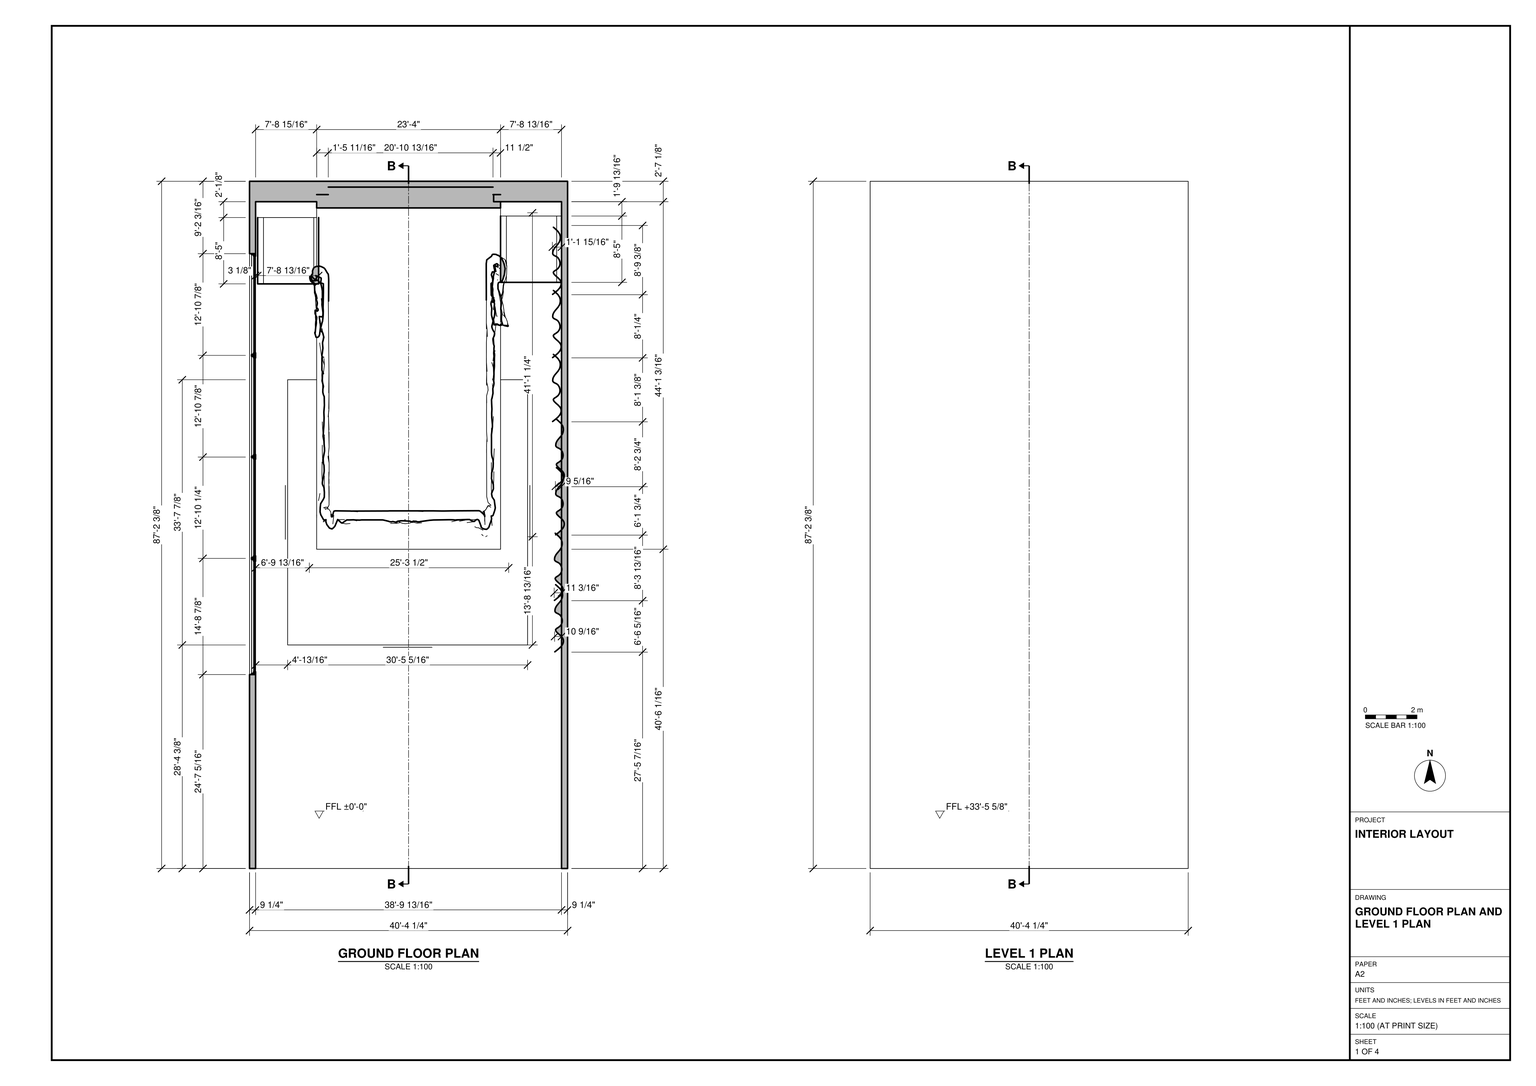
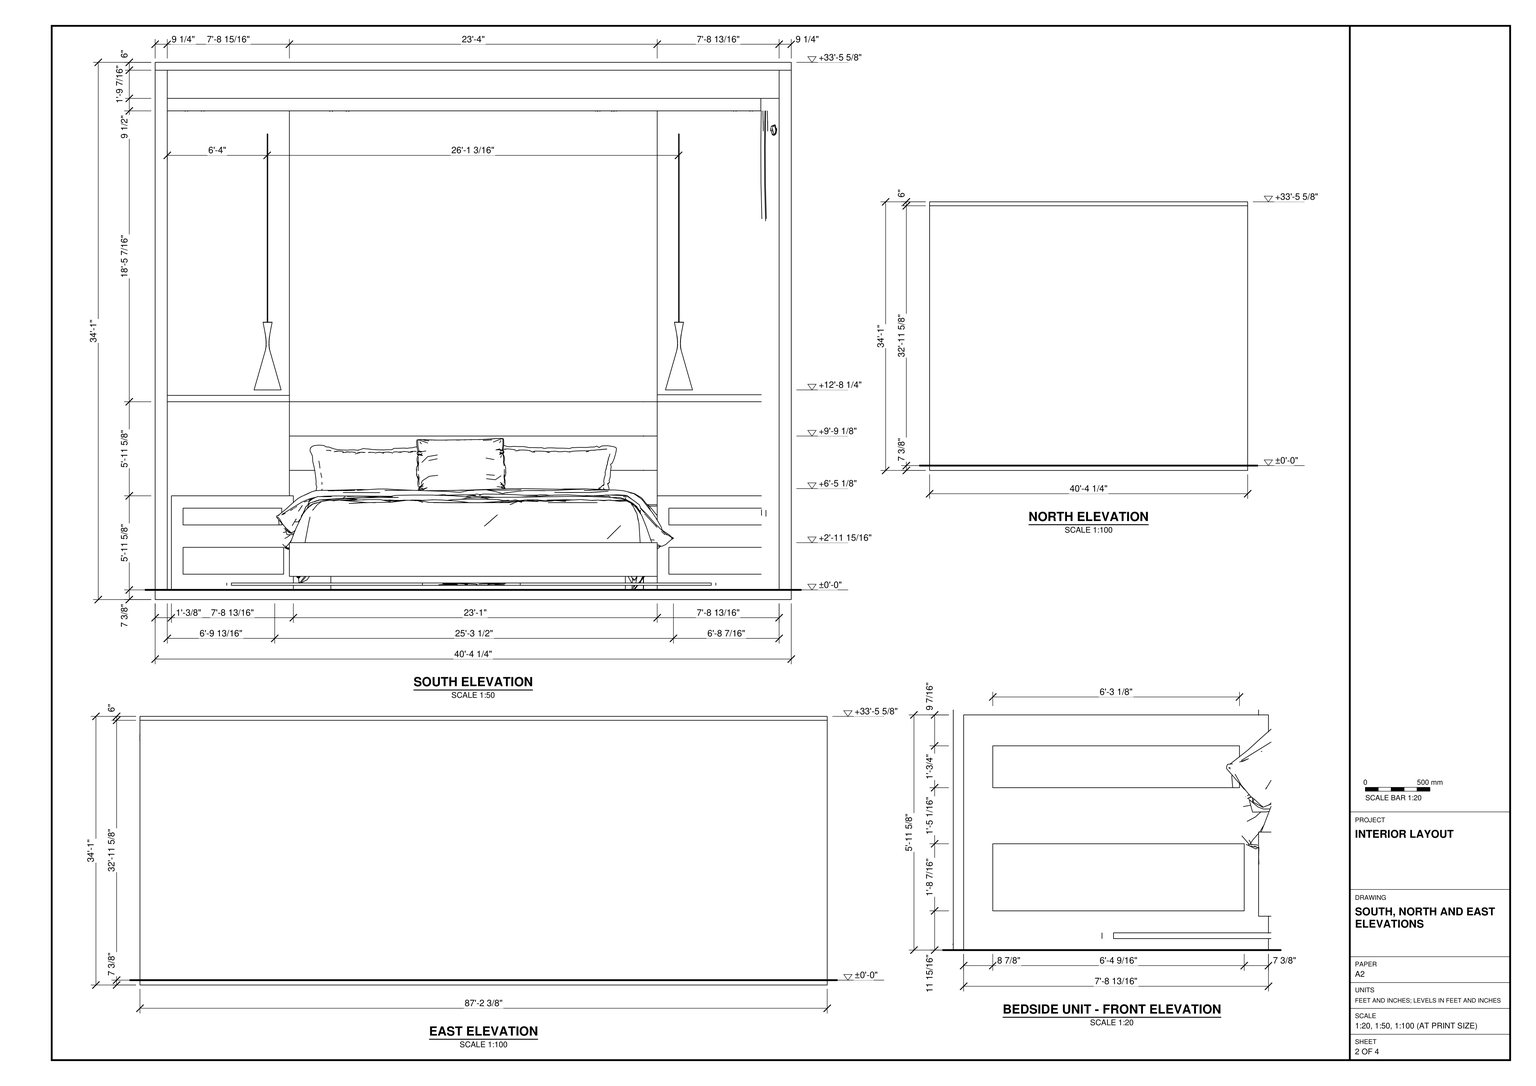
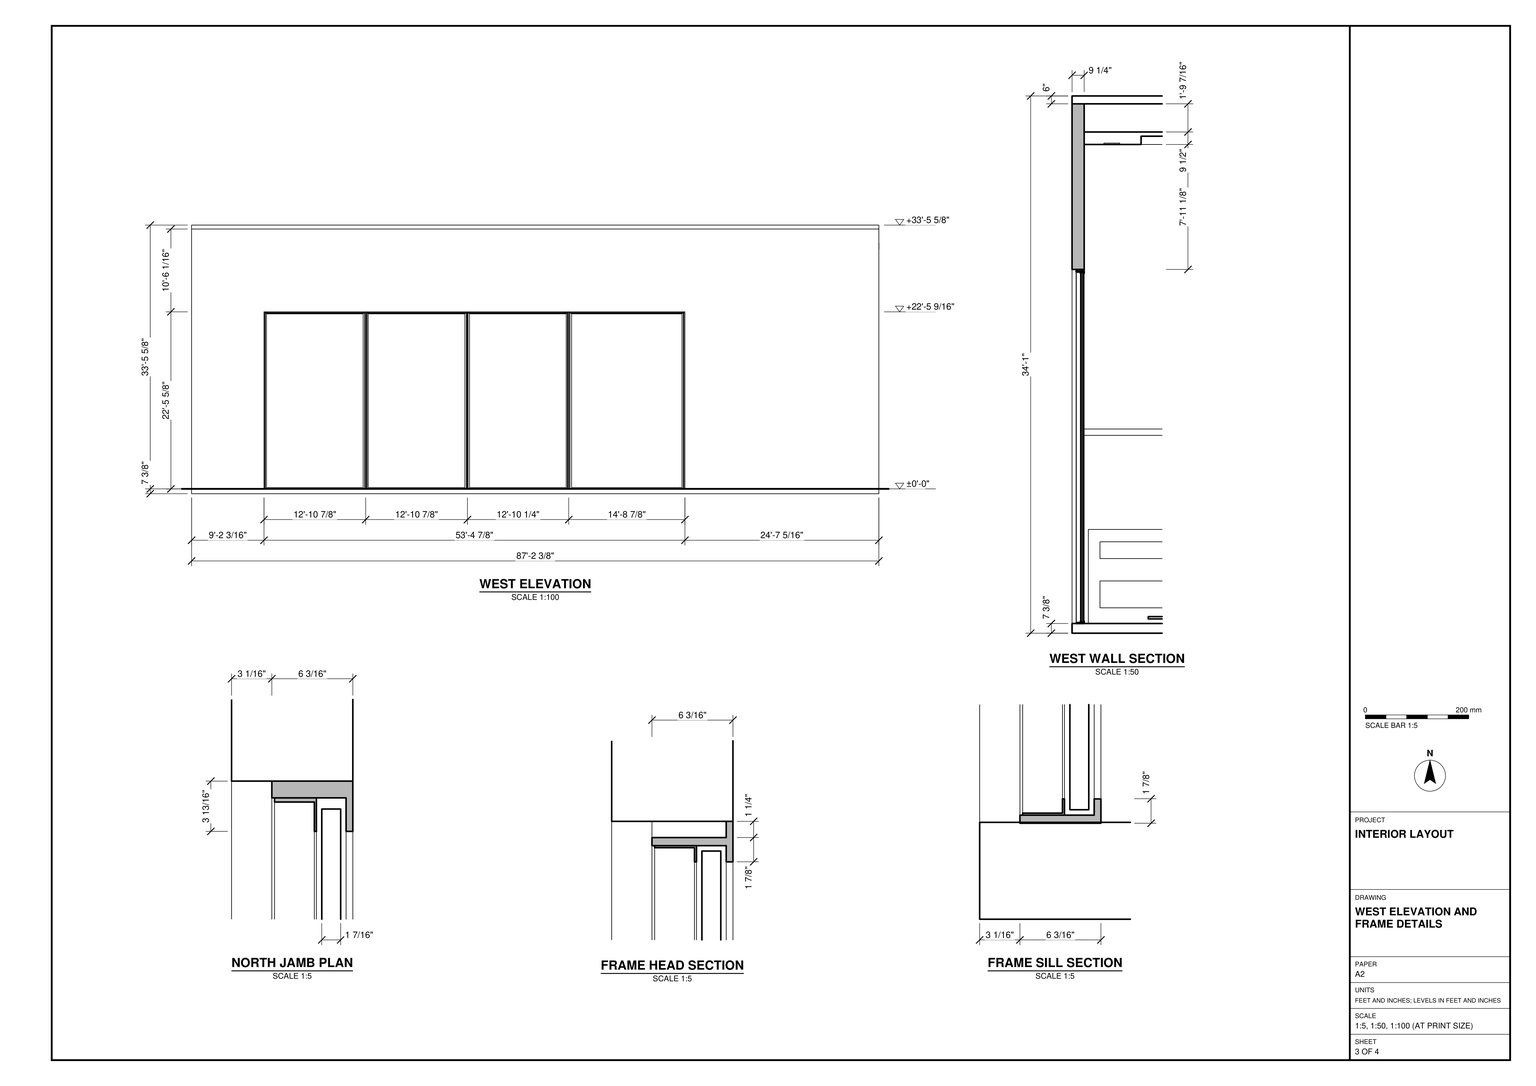
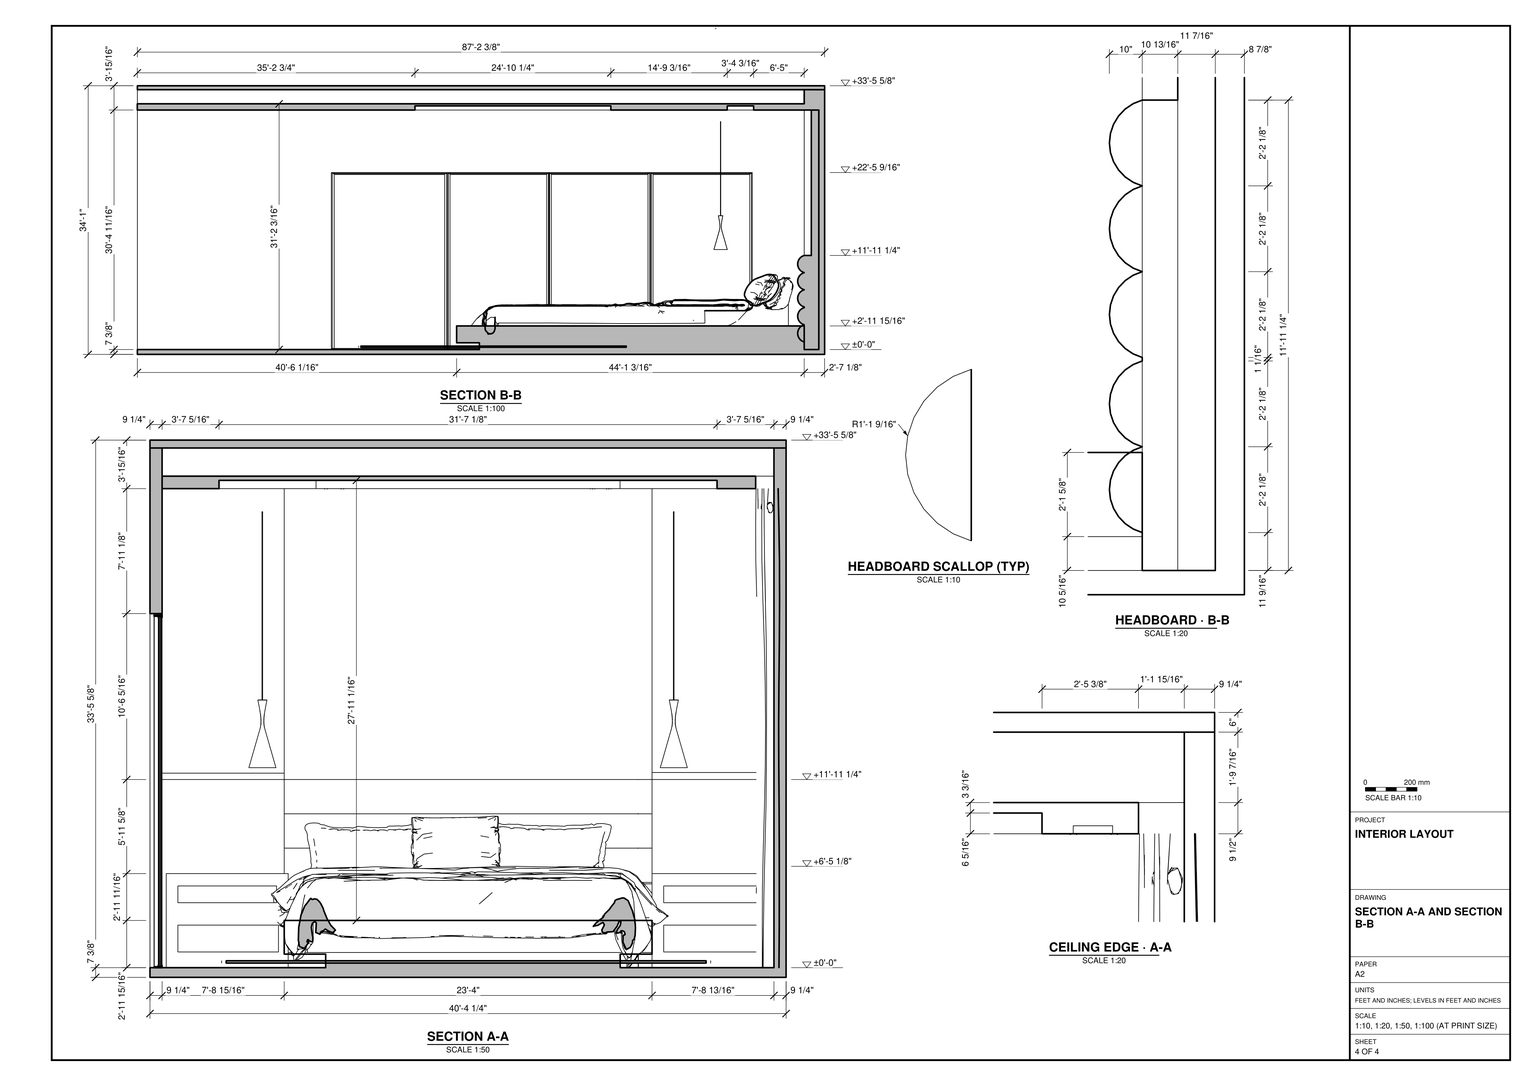
Build the bedroom interior in SketchUp from task_files/diagram_01.pdf. Work in feet and inches. The overall model is 40'-4 1/4" wide, 87'-2 1/2" long and 41'-4 3/8" high. Set the ground floor at ±0'-0" and Level 1 at +33'-5 5/8".

Model the floor slab, the two long side walls, the closed north end and the flat slab overhead. Leave the south end open as shown in plan. Follow the drawn wall thicknesses, including the 9 1/4" side walls. Fit the west wall opening with the sliding glazed panels. Use the west elevation for their spacing and the jamb, head and sill details for the frame.

Centre the platform bed against the north end with its foot toward the open floor area. Model the mattress, the panel behind the bed, the flanking ledges and the bedside storage units with their two stacked drawer fronts. Place the rug under the foot of the bed, the pendant lights above the bedside units and the curtain along the east side as shown. Decor and loose items may be any suitable library components.

Keep shell elements and individual furniture and joinery pieces in separate groups or components, and use components for repeated parts. Save one SketchUp model as output_files/bedroom_with_bedside_joinery_and_sliding_glazing.skp.

# SketchUp Ruby script. Lengths in inches.
U = 1.inch
M = Sketchup.active_model
def pt(a) = Geom::Point3d.new(a.map { |v| v * U })
def face(e, loops, mat)
  f = e.add_face(loops[0].map { |a| pt(a) })
  loops[1..].each { |l| e.add_face(l.map { |a| pt(a) }).erase! }
  f.material = f.back_material = mat if mat
  f
end
# faces: each face lists its corners as indices into pts; further lists are holes
def faces(e, pts, list, mat = nil) = list.each { |f| face(e, (f[0].is_a?(Array) ? f : [f]).map { |l| l.map { |i| pts[i] } }, mat) }
# xy, xz, yz: faces in a plane at the given z, y or x. An outline is a flat list of corners, or four numbers for a rectangle; further outlines are holes
def ring(l) = l.size == 4 ? [[l[0], l[1]], [l[2], l[1]], [l[2], l[3]], [l[0], l[3]]] : l.each_slice(2).to_a
def flat(e, list, mat, &to3) = list.each { |f| face(e, (f[0].is_a?(Array) ? f : [f]).map { |l| ring(l).map { |u, v| to3.(u, v) } }, mat) }
def xy(e, z, list, mat = nil) = flat(e, list, mat) { |x, y| [x, y, z] }
def xz(e, y, list, mat = nil) = flat(e, list, mat) { |x, z| [x, y, z] }
def yz(e, x, list, mat = nil) = flat(e, list, mat) { |y, z| [x, y, z] }
def lines(e, pts, list) = list.each { |a, b| e.add_line(pt(pts[a]), pt(pts[b])) }
# prism: a flat outline (further loops are holes) pulled along v
def prism(e, loops, v, mat = nil)
  f = face(e, loops, mat); d = Geom::Vector3d.new(v.map { |x| x * U })
  f.pushpull(f.normal.samedirection?(d) ? d.length : -d.length)
end
def box(e, o, s, mat = nil) = prism(e, [[o, [o[0] + s[0], o[1], o[2]], [o[0] + s[0], o[1] + s[1], o[2]], [o[0], o[1] + s[1], o[2]]]], [0, 0, s[2]], mat)
def at(x, y, z, deg = 0) = Geom::Transformation.translation(pt([x, y, z])) * Geom::Transformation.rotation(ORIGIN, Z_AXIS, deg.degrees)
def axes(o, x, y, z) = Geom::Transformation.new([*x, 0, *y, 0, *z, 0, *pt(o).to_a, 1])
def part(name) = M.definitions.add(name)
# library, detail: a bought-in or finely detailed component or shape, given as its bounding box
def library(name, o, s) = part(name).tap { |d| box(d.entities, o, s) }
def detail(e, o, s) = box(e.add_group.entities, o, s)
def put(e, d, t, mat = nil) = e.add_instance(d, t).tap { |i| i.material = mat if mat }
def group(e, t, mat = nil) = e.add_group.tap { |g| g.transformation = t; g.material = mat if mat }.entities
root = M.entities
M.materials.add("Glazing").color = [128, 128, 128]
M.materials["Glazing"].alpha = 0.05
M.materials.add("Material~3").color = [123, 113, 102]
M.materials.add("Powdercoating").color = [41, 44, 40]
M.materials.add("[0032_Moccasin]").color = [255, 228, 181]
M.materials.add("[Color M04]").color = [142, 142, 142]
M.materials.add("[Color M06]").color = [84, 84, 84]
M.materials.add("[Color M08]").color = [30, 30, 30]
M.materials.add("[Wood Cherry Original]").color = [135, 76, 37]
M.materials.add("[Wood Floor Dark]").color = [153, 94, 42]
M.materials.add("[Wood Floor]").color = [117, 79, 46]
M.materials.add("[Wood Veneer 01]").color = [119, 69, 36]
M.materials.add("bed 1").color = [202, 193, 182]
M.materials.add("rug").color = [176, 171, 170]
c1 = part("Group\#15")
xy(c1.entities,0,[[0,-55.94,0.71,45.94]])
xy(c1.entities,0.2,[[0,-55.94,0.47,45.94],[0.47,45.94,0.71,46.42]])
xy(c1.entities,2.36,[[0.47,-55.94,0.71,46.42]])
xz(c1.entities,-55.94,[[0,0,0.71,0,0.71,2.36,0.47,2.36,0.47,0.2,0,0.2]])
xz(c1.entities,45.94,[[0,0,0.71,0.2]])
xz(c1.entities,46.42,[[0.47,0.2,0.71,2.36]])
yz(c1.entities,0,[[-55.94,0,45.94,0.2]])
yz(c1.entities,0.47,[[-55.94,0.2,46.42,2.36]])
yz(c1.entities,0.71,[[-55.94,0,45.94,0,45.94,0.2,46.42,0.2,46.42,2.36,-55.94,2.36]])
c2 = part("Group\#7")
xy(c2.entities,0,[[0,-59.09,0.71,45.94]])
xy(c2.entities,0.2,[[0,-59.09,0.47,45.94],[0.47,45.94,0.71,46.42]])
xy(c2.entities,2.36,[[0.47,-59.09,0.71,46.42]])
xz(c2.entities,-59.09,[[0,0,0.71,0,0.71,2.36,0.47,2.36,0.47,0.2,0,0.2]])
xz(c2.entities,45.94,[[0,0,0.71,0.2]])
xz(c2.entities,46.42,[[0.47,0.2,0.71,2.36]])
yz(c2.entities,0,[[-59.09,0,45.94,0.2]])
yz(c2.entities,0.47,[[-59.09,0.2,46.42,2.36]])
yz(c2.entities,0.71,[[-59.09,0,45.94,0,45.94,0.2,46.42,0.2,46.42,2.36,-59.09,2.36]])
c3 = part("Group\#16")
prism(c3.entities,[[[0.47,-56.18,0.2],[0,-56.18,0.2],[0,-56.18,0],[0.71,-56.18,0],[0.71,-56.18,2.36],[0.47,-56.18,2.36]]],[0,28.68,0])
c4 = part("Group\#10")
box(c4.entities,[-0.73,0,0],[27.99,0.55,102.05])
c5 = part("Group\#18")
xy(c5.entities,0,[[0.47,-56.18,0.47,-55.47,0,-55.47,0,-28.21,1.18,-28.21,1.18,-56.18]])
xy(c5.entities,0.2,[[0.71,-56.18,1.18,-28.21],[0,-55.47,0.47,-28.21],[0.47,-28.21,0.71,-27.74]])
xy(c5.entities,2.36,[[0.47,-56.18,0.71,-27.74]])
xz(c5.entities,-56.18,[[0.47,0,1.18,0,1.18,0.2,0.71,0.2,0.71,2.36,0.47,2.36]])
xz(c5.entities,-55.47,[[0,0,0.47,0.2]])
xz(c5.entities,-28.21,[[0,0,1.18,0.2]])
xz(c5.entities,-27.74,[[0.47,0.2,0.71,2.36]])
yz(c5.entities,0,[[-55.47,0,-28.21,0.2]])
yz(c5.entities,0.47,[[-56.18,0,-55.47,0.2],[-56.18,0.2,-27.74,2.36]])
yz(c5.entities,0.71,[[-56.18,0.2,-27.74,2.36]])
yz(c5.entities,1.18,[[-56.18,0,-28.21,0.2]])
c6 = part("Group\#34")
xy(c6.entities,0,[[-20.45,0,7.76,1.22]])
xy(c6.entities,0.06,[[-20.39,0.06,7.7,1.22]])
xy(c6.entities,0.47,[[-19.98,0,7.28,0.06]])
xy(c6.entities,101.89,[[-19.98,0,7.28,0.06]])
xy(c6.entities,102.3,[[-20.39,0.06,7.7,1.22]])
xy(c6.entities,102.36,[[-20.45,0,7.76,1.22]])
xz(c6.entities,0,[[[-20.45,0,7.76,102.36],[-19.98,0.47,7.28,101.89]]])
xz(c6.entities,0.06,[[[-20.39,0.06,7.7,102.3],[-19.98,0.47,7.28,101.89]]])
xz(c6.entities,1.22,[[[-20.45,0,7.76,102.36],[-20.39,0.06,7.7,102.3]]])
yz(c6.entities,-20.45,[[0,0,1.22,102.36]])
yz(c6.entities,-20.39,[[0.06,0.06,1.22,102.3]])
yz(c6.entities,-19.98,[[0,0.47,0.06,101.89]])
yz(c6.entities,7.28,[[0,0.47,0.06,101.89]])
yz(c6.entities,7.7,[[0.06,0.06,1.22,102.3]])
yz(c6.entities,7.76,[[0,0,1.22,102.36]])
c7 = part("Group\#6")
put(c7.entities,c1,axes([27.97,0,7.875],[1,0,0],[0,0,-1],[0,1,0]),"Powdercoating")
put(c7.entities,c2,axes([0.71,0,6.8],[-1,0,0],[0,0,-0.97687],[0,1,0]),"Powdercoating")
put(c7.entities,c3,axes([-27.5,0,-38.07],[0,0,-1],[-1,0,0],[0,1,0]),"Powdercoating")
put(c7.entities,c4,at(1.12,0.35,-38.39),"Glazing")
put(c7.entities,c5,axes([-27.5,0,63.35],[0,0,1],[-1,0,0],[0,1,0]),"Powdercoating")
put(c7.entities,c6,at(20.6875,1.0625,-38.54),"Powdercoating")
c8 = part("Sliding glazed panels")
put(c8.entities,c7,at(-1.18,4.5,38.86))
g1 = group(c8.entities,at(84.74,4.5,38.86))
put(g1,c1,axes([-27.97,0,7.875],[-1,0,0],[0,0,-1],[0,1,0]),"Powdercoating")
put(g1,c2,axes([-0.71,0,6.8],[1,0,0],[0,0,-0.97687],[0,1,0]),"Powdercoating")
put(g1,c3,axes([27.5,0,-38.07],[0,0,-1],[1,0,0],[0,1,0]),"Powdercoating")
put(g1,c4,axes([-1.12,0.35,-38.39],[-1,0,0],[0,1,0],[0,0,1]),"Glazing")
put(g1,c5,axes([27.5,0,63.35],[0,0,1],[1,0,0],[0,1,0]),"Powdercoating")
put(g1,c6,axes([-20.6875,1.0625,-38.54],[-1,0,0],[0,1,0],[0,0,1]),"Powdercoating")
g2 = group(c8.entities,at(56.0625,4.5,38.86))
put(g2,c1,axes([-27.97,0,7.875],[-1,0,0],[0,0,-1],[0,1,0]),"Powdercoating")
put(g2,c3,axes([27.5,0,-38.07],[0,0,-1],[1,0,0],[0,1,0]),"Powdercoating")
put(g2,c4,axes([-1.12,0.35,-38.39],[-1,0,0],[0,1,0],[0,0,1]),"Glazing")
put(g2,c5,axes([27.5,0,63.35],[0,0,1],[1,0,0],[0,1,0]),"Powdercoating")
put(g2,c6,axes([-20.6875,1.0625,-38.54],[-1,0,0],[0,1,0],[0,0,1]),"Powdercoating")
g3 = group(g2,at(-0.71,0,6.8),"Powdercoating")
xy(g3,-45.34,[[0.47,0.2,0.71,2.36]])
xy(g3,-44.88,[[0,0,0.71,0.2]])
xy(g3,57.73,[[0,0,0.71,0,0.71,2.36,0.47,2.36,0.47,0.2,0,0.2]])
xz(g3,0,[[0,-44.88,0.71,57.73]])
xz(g3,0.2,[[0.47,-45.34,0.71,-44.88],[0,-44.88,0.47,57.73]])
xz(g3,2.36,[[0.47,-45.34,0.71,57.73]])
yz(g3,0,[[0,-44.88,0.2,57.73]])
yz(g3,0.47,[[0.2,-45.34,2.36,57.73]])
yz(g3,0.71,[[0.2,-45.34,2.36,-45.34,2.36,57.73,0,57.73,0,-44.88,0.2,-44.88]])
put(c8.entities,c7,axes([-33.94,4.5,38.86],[1.14218,0,0],[0,1,0],[0,0,1]))
c9 = part("sliding door")
put(c9.entities,c8,at(0,-4.5,-0.08))
c10 = library("3DGeom~4_Defintion",[362.52,-15.59,12.6],[288.85,70.11,1000])
c11 = library("rug",[-0.5,-0.5,0],[53.1875,58.7,0.25])
c12 = library("10 (1)",[26.65,-5.45,122.92],[1.37,1.38,0.36])
c13 = part("Group\#1")
xy(c13.entities,0,[[0,0,92.82,101]],"[Wood Cherry Original]")
xy(c13.entities,11.94,[[8.88,0,85.44,101]],"[Color M08]")
xy(c13.entities,32.38,[[8.88,0,85.44,101]],"[Wood Cherry Original]")
xy(c13.entities,49.45,[[8.87,0,83.99,101]],"[Color M08]")
xy(c13.entities,62.2,[[8.87,0,83.99,101]],"[Wood Cherry Original]")
xy(c13.entities,71.625,[[0,0,92.82,101]],"[Wood Cherry Original]")
xz(c13.entities,0,[[[0,0,92.82,71.625],[8.88,11.94,85.44,32.38],[8.87,49.45,83.99,62.2]]],"[Wood Cherry Original]")
xz(c13.entities,101,[[8.88,11.94,85.44,32.38],[8.87,49.45,83.99,62.2]],"[Color M08]")
yz(c13.entities,0,[[0,0,101,71.625]],"[Wood Cherry Original]")
yz(c13.entities,8.87,[[0,49.45,101,62.2]],"[Wood Cherry Original]")
yz(c13.entities,8.88,[[0,11.94,101,32.38]],"[Wood Cherry Original]")
yz(c13.entities,83.99,[[0,49.45,101,62.2]],"[Wood Cherry Original]")
yz(c13.entities,85.44,[[0,11.94,101,32.38]],"[Wood Cherry Original]")
yz(c13.entities,92.82,[[0,0,101,71.625]],"[Wood Cherry Original]")
c14 = library("skpD0DA",[-43.375,-44.17,6.95],[90.15,69.74,22.4])
c15 = library("Pillow mid",[-1042.59,1283.04,1394.37],[650.16,189.78,364.56])
c16 = library("Pillow mi0",[374.75,1266.66,1401.39],[641.67,174.72,385.96])
c17 = library("组\#9",[0,0,0],[17.22,12.51,16.85])
c18 = library("Grouper\#3",[0,0,0],[5.66,5.63,53.54])
xy(root,0,[[0,0.125,484.25,1046.5]])
xy(root,7.375,[[102.2,1015.39,371.64,1015.39,371.64,1026.21,370.7,1026.21,370.7,1037.64,119.88,1037.64,119.88,1026.21,102.2,1026.21],[371.64,1015.39,382.2,1026.21]])
xy(root,7.375,[[9.23,0.125,475.02,0.125,475.02,1015.39,357.95,1015.39,357.95,520.83,133.76,520.83,133.76,1015.39,9.23,1015.39,9.23,936.29,0,936.29,0,295.42,9.23,295.42]],"[Wood Floor Dark]")
xy(root,17.6875,[[102.2,486.21,133.76,1015.39],[133.76,486.21,133.76,520.83,357.95,520.83,357.95,500.08,382.2,500.08,382.2,486.21],[357.95,500.08,382.2,1015.39]])
xy(root,43.3125,[[102.2,486.21,382.2,486.21,382.2,1015.39,119.88,1015.39,119.88,1011.66,102.2,1011.66]],"[Wood Veneer 01]")
xy(root,150.62,[[102.2,1015.39,371.64,1026.21],[371.64,1015.39,382.2,1026.21]])
xy(root,276.9375,[[0,295.42,9.23,936.29]])
xy(root,372.05,[[119.88,1026.21,370.7,1037.64]])
xy(root,372.05,[[[9.23,0,9.23,1015.39,102.2,1015.39,102.2,1026.21,382.2,1026.21,382.2,1015.39,461.08,1015.39,461.08,0],[52.56,422.76,431.69,938.38],[342.69,1006.43,344.25,1006.63,345.69,1007.23,346.9375,1008.18,347.89,1009.43,348.49,1010.87,348.69,1012.43,348.49,1013.98,347.89,1015.43,346.9375,1016.67,345.69,1017.62,344.25,1018.22,342.69,1018.43,341.14,1018.22,339.69,1017.62,338.45,1016.67,337.5,1015.43,336.9,1013.98,336.69,1012.43,336.9,1010.87,337.5,1009.43,338.45,1008.18,339.69,1007.23,341.14,1006.63],[342.69,971.23,344.25,971.44,345.69,972.03,346.9375,972.99,347.89,974.23,348.49,975.68,348.69,977.23,348.49,978.78,347.89,980.23,346.9375,981.47,345.69,982.43,344.25,983.03,342.69,983.23,341.14,983.03,339.69,982.43,338.45,981.47,337.5,980.23,336.9,978.78,336.69,977.23,336.9,975.68,337.5,974.23,338.45,972.99,339.69,972.03,341.14,971.44],[447.2,804.63,448.76,804.84,450.2,805.4375,451.45,806.39,452.4,807.63,453,809.08,453.2,810.63,453,812.1875,452.4,813.63,451.45,814.875,450.2,815.83,448.76,816.43,447.2,816.63,445.65,816.43,444.2,815.83,442.96,814.875,442.01,813.63,441.41,812.1875,441.2,810.63,441.41,809.08,442.01,807.63,442.96,806.39,444.2,805.4375,445.65,804.84],[30.24,804.63,31.79,804.84,33.24,805.4375,34.48,806.39,35.44,807.63,36.03,809.08,36.24,810.63,36.03,812.1875,35.44,813.63,34.48,814.875,33.24,815.83,31.79,816.43,30.24,816.63,28.6875,816.43,27.24,815.83,26,814.875,25.04,813.63,24.44,812.1875,24.24,810.63,24.44,809.08,25.04,807.63,26,806.39,27.24,805.4375,28.6875,804.84],[141.05,999.02,142.58,999.31,144,999.99,145.18,1001.01,146.07,1002.3,146.58,1003.78,146.7,1005.34,146.41,1006.88,145.73,1008.29,144.71,1009.48,143.42,1010.36,141.9375,1010.88,140.375,1011,138.84,1010.71,137.43,1010.03,136.24,1009.01,135.36,1007.71,134.84,1006.23,134.72,1004.67,135.01,1003.13,135.69,1001.72,136.71,1000.53,138,999.65,139.48,999.13],[140.71,963.9375,142.24,964.14,143.66,964.73,144.88,965.66,145.8125,966.88,146.4,968.3,146.6,969.83,146.4,971.35,145.8125,972.78,144.88,974,143.66,974.93,142.24,975.52,140.71,975.72,139.19,975.52,137.76,974.93,136.54,974,135.61,972.78,135.02,971.35,134.82,969.83,135.02,968.3,135.61,966.88,136.54,965.66,137.76,964.73,139.19,964.14]],[126.41,721,357.84,898.21]],"[Wood Cherry Original]")
xy(root,373.12,[[30.24,804.63,28.6875,804.84,27.24,805.4375,26,806.39,25.04,807.63,24.44,809.08,24.24,810.63,24.44,812.1875,25.04,813.63,26,814.875,27.24,815.83,28.6875,816.43,30.24,816.63,31.79,816.43,33.24,815.83,34.48,814.875,35.44,813.63,36.03,812.1875,36.24,810.63,36.03,809.08,35.44,807.63,34.48,806.39,33.24,805.4375,31.79,804.84],[140.71,963.9375,139.19,964.14,137.76,964.73,136.54,965.66,135.61,966.88,135.02,968.3,134.82,969.83,135.02,971.35,135.61,972.78,136.54,974,137.76,974.93,139.19,975.52,140.71,975.72,142.24,975.52,143.66,974.93,144.88,974,145.8125,972.78,146.4,971.35,146.6,969.83,146.4,968.3,145.8125,966.88,144.88,965.66,143.66,964.73,142.24,964.14],[342.69,971.23,341.14,971.44,339.69,972.03,338.45,972.99,337.5,974.23,336.9,975.68,336.69,977.23,336.9,978.78,337.5,980.23,338.45,981.47,339.69,982.43,341.14,983.03,342.69,983.23,344.25,983.03,345.69,982.43,346.9375,981.47,347.89,980.23,348.49,978.78,348.69,977.23,348.49,975.68,347.89,974.23,346.9375,972.99,345.69,972.03,344.25,971.44],[141.05,999.02,139.48,999.13,138,999.65,136.71,1000.53,135.69,1001.72,135.01,1003.13,134.72,1004.67,134.84,1006.23,135.36,1007.71,136.24,1009.01,137.43,1010.03,138.84,1010.71,140.375,1011,141.9375,1010.88,143.42,1010.36,144.71,1009.48,145.73,1008.29,146.41,1006.88,146.7,1005.34,146.58,1003.78,146.07,1002.3,145.18,1001.01,144,999.99,142.58,999.31]],"[Wood Cherry Original]")
xy(root,374.49,[[447.2,804.63,445.65,804.84,444.2,805.4375,442.96,806.39,442.01,807.63,441.41,809.08,441.2,810.63,441.41,812.1875,442.01,813.63,442.96,814.875,444.2,815.83,445.65,816.43,447.2,816.63,448.76,816.43,450.2,815.83,451.45,814.875,452.4,813.63,453,812.1875,453.2,810.63,453,809.08,452.4,807.63,451.45,806.39,450.2,805.4375,448.76,804.84]],"[Wood Cherry Original]")
xy(root,374.55,[[342.69,1006.43,341.14,1006.63,339.69,1007.23,338.45,1008.18,337.5,1009.43,336.9,1010.87,336.69,1012.43,336.9,1013.98,337.5,1015.43,338.45,1016.67,339.69,1017.62,341.14,1018.22,342.69,1018.43,344.25,1018.22,345.69,1017.62,346.9375,1016.67,347.89,1015.43,348.49,1013.98,348.69,1012.43,348.49,1010.87,347.89,1009.43,346.9375,1008.18,345.69,1007.23,344.25,1006.63]],"[Wood Cherry Original]")
xy(root,378.37,[[[52.56,422.76,431.69,938.38],[126.41,721,357.84,898.21]]],"[Wood Floor]")
xy(root,381.55,[[9.23,0,461.08,1015.39]])
xy(root,403,[[0,0.125,0,1046.5,484.25,1046.5,484.25,0.125,475.02,0.125,475.02,1015.39,9.23,1015.39,9.23,0.125],[9.23,0.125,475.02,1015.39]])
xy(root,409,[[0,0.125,484.25,1046.5]])
xz(root,0,[[9.23,372.05,461.08,381.55]])
xz(root,0.125,[[0,0,484.25,0,484.25,403,475.02,403,475.02,7.375,9.23,7.375,9.23,403,0,403],[0,403,484.25,409]])
xz(root,295.42,[[0,7.375,9.23,276.9375]])
xz(root,422.76,[[52.56,372.05,431.69,378.37]])
xz(root,486.21,[[102.2,17.6875,382.2,43.3125]],"[Wood Veneer 01]")
xz(root,520.83,[[133.76,7.375,357.95,17.6875]])
xz(root,721,[[126.41,372.05,357.84,378.37]],"[Wood Floor]")
xz(root,898.21,[[126.41,372.05,357.84,378.37]])
xz(root,936.29,[[0,7.375,9.23,276.9375]])
xz(root,938.38,[[52.56,372.05,431.69,378.37]],"[Wood Floor]")
xz(root,1015.39,[[102.2,7.375,133.76,17.6875],[133.76,7.375,133.76,17.6875,102.2,17.6875,102.2,18.93,371.64,18.93,371.64,17.6875,357.95,17.6875,357.95,7.375],[357.95,7.375,371.64,17.6875],[371.64,7.375,371.82,17.6875],[371.82,7.375,382.2,17.6875],
  [371.64,17.6875,382.2,18.93],[102.2,18.93,119.88,43.3125],[119.88,18.93,370.7,43.3125],[370.7,18.93,371.64,43.3125],[371.64,18.93,382.2,43.3125],
  [102.2,43.3125,119.88,45.05],[370.7,43.3125,371.64,45.05],[371.64,43.3125,382.2,45.05],[371.64,45.05,382.2,71.18],[102.2,71.18,371.64,72.25],
  [371.64,71.18,382.2,72.25],[371.64,72.25,382.2,98.37],[371.64,98.37,382.2,124.5],[371.64,124.5,382.2,150.62],[9.23,381.55,475.02,403]])
xz(root,1015.39,[[382.2,150.62,475.02,155.95]],"[Wood Cherry Original]")
xz(root,1015.39,[[9.23,7.375,102.2,150.62],[382.2,7.375,475.02,150.62],[9.23,150.62,102.2,155.45],[9.23,155.45,102.2,372.05],[382.2,155.95,475.02,155.95,475.02,381.55,461.08,381.55,461.08,372.05,382.2,372.05]],"[Wood Veneer 01]")
xz(root,1026.21,[[102.2,7.375,119.88,150.62],[370.7,7.375,371.64,150.62],[371.64,7.375,382.2,150.62]])
xz(root,1026.21,[[102.2,150.62,382.2,372.05]],"[Wood Floor]")
xz(root,1037.64,[[119.88,7.375,370.7,372.05]])
xz(root,1046.5,[[0,0,484.25,403],[0,403,484.25,409]])
yz(root,0,[[[0.125,0,1046.5,403],[295.42,7.375,936.29,276.9375]],[0.125,403,1046.5,409]])
yz(root,9.23,[[0,372.05,0.125,381.55],[0.125,372.05,1015.39,381.55],[0.125,381.55,1015.39,403]])
yz(root,9.23,[[0.125,7.375,295.42,7.375,295.42,276.9375,936.29,276.9375,936.29,7.375,1015.39,7.375,1015.39,372.05,0.125,372.05]],"[0032_Moccasin]")
yz(root,52.56,[[422.76,372.05,938.38,378.37]],"[Wood Floor]")
yz(root,102.2,[[1015.39,45.05,1012.65,46.12,1010.21,47.76,1008.18,49.89,1006.66,52.4,1005.71,55.1875,1005.39,58.11,1005.71,61.04,1006.66,63.82,1008.18,66.34,1010.21,68.47,1012.65,70.1,1015.39,71.18],[1015.39,72.25,1012.65,73.32,1010.21,74.96,1008.18,77.08,1006.66,79.6,1005.71,82.39,1005.39,85.31,1005.71,88.23,1006.66,91.02,1008.18,93.53,1010.21,95.66,1012.65,97.3,1015.39,98.37],[1015.39,98.37,1012.65,99.44,1010.21,101.08,1008.18,103.21,1006.66,105.73,1005.71,108.51,1005.39,111.43,1005.71,114.36,1006.66,117.14,1008.18,119.66,1010.21,121.79,1012.65,123.43,1015.39,124.5],[1015.39,124.5,1012.65,125.57,1010.21,127.21,1008.18,129.33,1006.66,131.85,1005.71,134.64,1005.39,137.56,1005.71,140.48,1006.66,143.27,1008.18,145.78,1010.21,147.91,1012.65,149.55,1015.39,150.62],[1015.39,150.62,1026.21,372.05]])
yz(root,102.2,[[486.21,17.6875,486.21,43.3125,1011.66,43.3125,1010.21,42.34,1008.18,40.21,1006.66,37.7,1005.71,34.91,1005.39,31.99,1005.71,29.0625,1006.66,26.28,1008.18,23.76,1010.21,21.64,1012.65,20,1015.39,18.93,1015.39,17.6875]],"[Wood Cherry Original]")
yz(root,119.88,[[1015.39,18.93,1012.65,20,1010.21,21.64,1008.18,23.76,1006.66,26.28,1005.71,29.0625,1005.39,31.99,1005.71,34.91,1006.66,37.7,1008.18,40.21,1010.21,42.34,1011.66,43.3125,1015.39,43.3125],[1011.66,43.3125,1012.65,43.98,1015.39,45.05,1015.39,43.3125]])
yz(root,126.41,[[721,372.05,898.21,378.37]])
yz(root,133.76,[[520.83,7.375,1015.39,17.6875]])
yz(root,357.84,[[721,372.05,898.21,378.37]])
yz(root,357.95,[[520.83,7.375,1015.39,17.6875]])
yz(root,370.7,[[1015.39,18.93,1015.39,45.05,1012.65,43.98,1010.21,42.34,1008.18,40.21,1006.66,37.7,1005.71,34.91,1005.39,31.99,1005.71,29.0625,1006.66,26.28,1008.18,23.76,1010.21,21.64,1012.65,20]])
yz(root,371.64,[[1015.39,7.375,1026.21,150.62]])
yz(root,382.2,[[1015.39,45.05,1015.39,71.18,1012.65,70.1,1010.21,68.47,1008.18,66.34,1006.66,63.82,1005.71,61.04,1005.39,58.11,1005.71,55.1875,1006.66,52.4,1008.18,49.89,1010.21,47.76,1012.65,46.12],[1015.39,72.25,1015.39,98.37,1012.65,97.3,1010.21,95.66,1008.18,93.53,1006.66,91.02,1005.71,88.23,1005.39,85.31,1005.71,82.39,1006.66,79.6,1008.18,77.08,1010.21,74.96,1012.65,73.32],[1015.39,98.37,1015.39,124.5,1012.65,123.43,1010.21,121.79,1008.18,119.66,1006.66,117.14,1005.71,114.36,1005.39,111.43,1005.71,108.51,1006.66,105.73,1008.18,103.21,1010.21,101.08,1012.65,99.44],[1015.39,124.5,1015.39,150.62,1012.65,149.55,1010.21,147.91,1008.18,145.78,1006.66,143.27,1005.71,140.48,1005.39,137.56,1005.71,134.64,1006.66,131.85,1008.18,129.33,1010.21,127.21,1012.65,125.57],[1015.39,150.62,1026.21,372.05]])
yz(root,382.2,[[486.21,17.6875,1015.39,43.3125]],"[Wood Cherry Original]")
yz(root,431.69,[[422.76,372.05,938.38,378.37]],"[Wood Floor]")
yz(root,461.08,[[0,372.05,1015.39,381.55]])
yz(root,475.02,[[0.125,7.375,1015.39,381.55],[0.125,381.55,1015.39,403]])
yz(root,484.25,[[0.125,0,1046.5,403],[0.125,403,1046.5,409]])
p = [[119.88,1012.65,20],[119.88,1015.39,18.93],[102.2,1015.39,18.93],[102.2,1012.65,20],[370.7,1015.39,18.93],[370.7,1012.65,20],
  [119.88,1010.21,21.64],[102.2,1010.21,21.64],[370.7,1010.21,21.64],[119.88,1008.18,23.76],[102.2,1008.18,23.76],[370.7,1008.18,23.76],
  [119.88,1006.66,26.28],[102.2,1006.66,26.28],[370.7,1006.66,26.28],[119.88,1005.71,29.0625],[102.2,1005.71,29.0625],[370.7,1005.71,29.0625],
  [119.88,1005.39,31.99],[102.2,1005.39,31.99],[370.7,1005.39,31.99],[119.88,1005.71,34.91],[102.2,1005.71,34.91],[370.7,1005.71,34.91],
  [119.88,1006.66,37.7],[102.2,1006.66,37.7],[370.7,1006.66,37.7],[119.88,1008.18,40.21],[102.2,1008.18,40.21],[370.7,1008.18,40.21],
  [119.88,1010.21,42.34],[102.2,1010.21,42.34],[370.7,1010.21,42.34],[119.88,1011.66,43.3125],[102.2,1011.66,43.3125],[119.88,1012.65,43.98],
  [370.7,1012.65,43.98],[119.88,1015.39,45.05],[370.7,1015.39,45.05],[382.2,1012.65,46.12],[102.2,1012.65,46.12],[102.2,1015.39,45.05],
  [371.64,1015.39,45.05],[382.2,1015.39,45.05],[382.2,1010.21,47.76],[102.2,1010.21,47.76],[382.2,1008.18,49.89],[102.2,1008.18,49.89],
  [382.2,1006.66,52.4],[102.2,1006.66,52.4],[382.2,1005.71,55.1875],[102.2,1005.71,55.1875],[382.2,1005.39,58.11],[102.2,1005.39,58.11],
  [382.2,1005.71,61.04],[102.2,1005.71,61.04],[382.2,1006.66,63.82],[102.2,1006.66,63.82],[382.2,1008.18,66.34],[102.2,1008.18,66.34],
  [382.2,1010.21,68.47],[102.2,1010.21,68.47],[382.2,1012.65,70.1],[102.2,1012.65,70.1],[371.64,1015.39,71.18],[102.2,1015.39,71.18],
  [382.2,1015.39,71.18],[102.2,1012.65,73.32],[102.2,1015.39,72.25],[371.64,1015.39,72.25],[382.2,1015.39,72.25],[382.2,1012.65,73.32],
  [102.2,1010.21,74.96],[382.2,1010.21,74.96],[102.2,1008.18,77.08],[382.2,1008.18,77.08],[102.2,1006.66,79.6],[382.2,1006.66,79.6],
  [102.2,1005.71,82.39],[382.2,1005.71,82.39],[102.2,1005.39,85.31],[382.2,1005.39,85.31],[102.2,1005.71,88.23],[382.2,1005.71,88.23],
  [102.2,1006.66,91.02],[382.2,1006.66,91.02],[102.2,1008.18,93.53],[382.2,1008.18,93.53],[102.2,1010.21,95.66],[382.2,1010.21,95.66],
  [102.2,1012.65,97.3],[382.2,1012.65,97.3],[102.2,1015.39,98.37],[382.2,1015.39,98.37],[371.64,1015.39,98.37],[382.2,1012.65,99.44],
  [102.2,1012.65,99.44],[382.2,1010.21,101.08],[102.2,1010.21,101.08],[382.2,1008.18,103.21],[102.2,1008.18,103.21],[382.2,1006.66,105.73],
  [102.2,1006.66,105.73],[382.2,1005.71,108.51],[102.2,1005.71,108.51],[382.2,1005.39,111.43],[102.2,1005.39,111.43],[382.2,1005.71,114.36],
  [102.2,1005.71,114.36],[382.2,1006.66,117.14],[102.2,1006.66,117.14],[382.2,1008.18,119.66],[102.2,1008.18,119.66],[382.2,1010.21,121.79],
  [102.2,1010.21,121.79],[382.2,1012.65,123.43],[102.2,1012.65,123.43],[371.64,1015.39,124.5],[102.2,1015.39,124.5],[382.2,1015.39,124.5],
  [382.2,1012.65,125.57],[102.2,1012.65,125.57],[382.2,1010.21,127.21],[102.2,1010.21,127.21],[382.2,1008.18,129.33],[102.2,1008.18,129.33],
  [382.2,1006.66,131.85],[102.2,1006.66,131.85],[382.2,1005.71,134.64],[102.2,1005.71,134.64],[382.2,1005.39,137.56],[102.2,1005.39,137.56],
  [382.2,1005.71,140.48],[102.2,1005.71,140.48],[382.2,1006.66,143.27],[102.2,1006.66,143.27],[382.2,1008.18,145.78],[102.2,1008.18,145.78],
  [382.2,1010.21,147.91],[102.2,1010.21,147.91],[382.2,1012.65,149.55],[102.2,1012.65,149.55],[371.64,1015.39,150.62],[102.2,1015.39,150.62],
  [382.2,1015.39,150.62],[30.24,804.63,372.05],[28.6875,804.84,372.05],[28.6875,804.84,373.12],[30.24,804.63,373.12],[31.79,804.84,372.05],
  [31.79,804.84,373.12],[447.2,804.63,372.05],[445.65,804.84,372.05],[445.65,804.84,374.49],[447.2,804.63,374.49],[448.76,804.84,372.05],
  [448.76,804.84,374.49],[27.24,805.4375,372.05],[27.24,805.4375,373.12],[33.24,805.4375,372.05],[33.24,805.4375,373.12],[444.2,805.4375,372.05],
  [444.2,805.4375,374.49],[450.2,805.4375,372.05],[450.2,805.4375,374.49],[26,806.39,372.05],[26,806.39,373.12],[34.48,806.39,372.05],
  [34.48,806.39,373.12],[442.96,806.39,372.05],[442.96,806.39,374.49],[451.45,806.39,372.05],[451.45,806.39,374.49],[25.04,807.63,372.05],
  [25.04,807.63,373.12],[35.44,807.63,372.05],[35.44,807.63,373.12],[442.01,807.63,372.05],[442.01,807.63,374.49],[452.4,807.63,372.05],
  [452.4,807.63,374.49],[24.44,809.08,372.05],[24.44,809.08,373.12],[36.03,809.08,372.05],[36.03,809.08,373.12],[441.41,809.08,372.05],
  [441.41,809.08,374.49],[453,809.08,372.05],[453,809.08,374.49],[24.24,810.63,372.05],[24.24,810.63,373.12],[36.24,810.63,372.05],
  [36.24,810.63,373.12],[441.2,810.63,372.05],[441.2,810.63,374.49],[453.2,810.63,372.05],[453.2,810.63,374.49],[24.44,812.1875,372.05],
  [24.44,812.1875,373.12],[36.03,812.1875,372.05],[36.03,812.1875,373.12],[441.41,812.1875,372.05],[441.41,812.1875,374.49],[453,812.1875,372.05],
  [453,812.1875,374.49],[25.04,813.63,372.05],[25.04,813.63,373.12],[35.44,813.63,372.05],[35.44,813.63,373.12],[442.01,813.63,372.05],
  [442.01,813.63,374.49],[452.4,813.63,372.05],[452.4,813.63,374.49],[26,814.875,372.05],[26,814.875,373.12],[34.48,814.875,372.05],
  [34.48,814.875,373.12],[442.96,814.875,372.05],[442.96,814.875,374.49],[451.45,814.875,372.05],[451.45,814.875,374.49],[27.24,815.83,372.05],
  [27.24,815.83,373.12],[33.24,815.83,372.05],[33.24,815.83,373.12],[444.2,815.83,372.05],[444.2,815.83,374.49],[450.2,815.83,372.05],
  [450.2,815.83,374.49],[28.6875,816.43,372.05],[28.6875,816.43,373.12],[31.79,816.43,372.05],[31.79,816.43,373.12],[445.65,816.43,372.05],
  [445.65,816.43,374.49],[448.76,816.43,372.05],[448.76,816.43,374.49],[30.24,816.63,372.05],[30.24,816.63,373.12],[447.2,816.63,372.05],
  [447.2,816.63,374.49],[140.71,963.9375,372.05],[139.19,964.14,372.05],[139.19,964.14,373.12],[140.71,963.9375,373.12],[142.24,964.14,372.05],
  [142.24,964.14,373.12],[137.76,964.73,372.05],[137.76,964.73,373.12],[143.66,964.73,372.05],[143.66,964.73,373.12],[136.54,965.66,372.05],
  [136.54,965.66,373.12],[144.88,965.66,372.05],[144.88,965.66,373.12],[135.61,966.88,372.05],[135.61,966.88,373.12],[145.8125,966.88,372.05],
  [145.8125,966.88,373.12],[135.02,968.3,372.05],[135.02,968.3,373.12],[146.4,968.3,372.05],[146.4,968.3,373.12],[134.82,969.83,372.05],
  [134.82,969.83,373.12],[146.6,969.83,372.05],[146.6,969.83,373.12],[135.02,971.35,372.05],[135.02,971.35,373.12],[146.4,971.35,372.05],
  [146.4,971.35,373.12],[342.69,971.23,372.05],[341.14,971.44,372.05],[341.14,971.44,373.12],[342.69,971.23,373.12],[344.25,971.44,372.05],
  [344.25,971.44,373.12],[135.61,972.78,372.05],[135.61,972.78,373.12],[145.8125,972.78,372.05],[145.8125,972.78,373.12],[339.69,972.03,372.05],
  [339.69,972.03,373.12],[345.69,972.03,372.05],[345.69,972.03,373.12],[338.45,972.99,372.05],[338.45,972.99,373.12],[346.9375,972.99,372.05],
  [346.9375,972.99,373.12],[136.54,974,372.05],[136.54,974,373.12],[144.88,974,372.05],[144.88,974,373.12],[337.5,974.23,372.05],
  [337.5,974.23,373.12],[347.89,974.23,372.05],[347.89,974.23,373.12],[137.76,974.93,372.05],[137.76,974.93,373.12],[143.66,974.93,372.05],
  [143.66,974.93,373.12],[336.9,975.68,372.05],[336.9,975.68,373.12],[348.49,975.68,372.05],[348.49,975.68,373.12],[139.19,975.52,372.05],
  [139.19,975.52,373.12],[142.24,975.52,372.05],[142.24,975.52,373.12],[140.71,975.72,372.05],[140.71,975.72,373.12],[336.69,977.23,372.05],
  [336.69,977.23,373.12],[348.69,977.23,372.05],[348.69,977.23,373.12],[336.9,978.78,372.05],[336.9,978.78,373.12],[348.49,978.78,372.05],
  [348.49,978.78,373.12],[337.5,980.23,372.05],[337.5,980.23,373.12],[347.89,980.23,372.05],[347.89,980.23,373.12],[338.45,981.47,372.05],
  [338.45,981.47,373.12],[346.9375,981.47,372.05],[346.9375,981.47,373.12],[339.69,982.43,372.05],[339.69,982.43,373.12],[345.69,982.43,372.05],
  [345.69,982.43,373.12],[341.14,983.03,372.05],[341.14,983.03,373.12],[344.25,983.03,372.05],[344.25,983.03,373.12],[342.69,983.23,372.05],
  [342.69,983.23,373.12],[141.05,999.02,372.05],[139.48,999.13,372.05],[139.48,999.13,373.12],[141.05,999.02,373.12],[142.58,999.31,372.05],
  [142.58,999.31,373.12],[138,999.65,372.05],[138,999.65,373.12],[144,999.99,372.05],[144,999.99,373.12],[136.71,1000.53,372.05],
  [136.71,1000.53,373.12],[145.18,1001.01,372.05],[145.18,1001.01,373.12],[135.69,1001.72,372.05],[135.69,1001.72,373.12],[146.07,1002.3,372.05],
  [146.07,1002.3,373.12],[135.01,1003.13,372.05],[135.01,1003.13,373.12],[146.58,1003.78,372.05],[146.58,1003.78,373.12],[134.72,1004.67,372.05],
  [134.72,1004.67,373.12],[146.7,1005.34,372.05],[146.7,1005.34,373.12],[134.84,1006.23,372.05],[134.84,1006.23,373.12],[146.41,1006.88,372.05],
  [146.41,1006.88,373.12],[135.36,1007.71,372.05],[135.36,1007.71,373.12],[342.69,1006.43,372.05],[341.14,1006.63,372.05],[341.14,1006.63,374.55],
  [342.69,1006.43,374.55],[344.25,1006.63,372.05],[344.25,1006.63,374.55],[339.69,1007.23,372.05],[339.69,1007.23,374.55],[345.69,1007.23,372.05],
  [345.69,1007.23,374.55],[145.73,1008.29,372.05],[145.73,1008.29,373.12],[338.45,1008.18,372.05],[338.45,1008.18,374.55],[346.9375,1008.18,372.05],
  [346.9375,1008.18,374.55],[136.24,1009.01,372.05],[136.24,1009.01,373.12],[337.5,1009.43,372.05],[337.5,1009.43,374.55],[347.89,1009.43,372.05],
  [347.89,1009.43,374.55],[144.71,1009.48,372.05],[144.71,1009.48,373.12],[137.43,1010.03,372.05],[137.43,1010.03,373.12],[336.9,1010.87,372.05],
  [336.9,1010.87,374.55],[348.49,1010.87,372.05],[348.49,1010.87,374.55],[143.42,1010.36,372.05],[143.42,1010.36,373.12],[138.84,1010.71,372.05],
  [138.84,1010.71,373.12],[141.9375,1010.88,372.05],[141.9375,1010.88,373.12],[140.375,1011,372.05],[140.375,1011,373.12],[336.69,1012.43,372.05],
  [336.69,1012.43,374.55],[348.69,1012.43,372.05],[348.69,1012.43,374.55],[336.9,1013.98,372.05],[336.9,1013.98,374.55],[348.49,1013.98,372.05],
  [348.49,1013.98,374.55],[337.5,1015.43,372.05],[337.5,1015.43,374.55],[347.89,1015.43,372.05],[347.89,1015.43,374.55],[338.45,1016.67,372.05],
  [338.45,1016.67,374.55],[346.9375,1016.67,372.05],[346.9375,1016.67,374.55],[339.69,1017.62,372.05],[339.69,1017.62,374.55],[345.69,1017.62,372.05],
  [345.69,1017.62,374.55],[341.14,1018.22,372.05],[341.14,1018.22,374.55],[344.25,1018.22,372.05],[344.25,1018.22,374.55],[342.69,1018.43,372.05],
  [342.69,1018.43,374.55]]
faces(root,p,[[0,1,2,3],[0,1,4,5],[6,0,3,7],[6,0,5,8],[9,6,7,10],[9,6,8,11],[12,9,10,13],[12,9,11,14],
  [15,12,13,16],[15,12,14,17],[18,15,16,19],[18,15,17,20],[21,18,19,22],[21,18,20,23],[24,21,22,25],[24,21,23,26],
  [27,24,25,28],[27,24,26,29],[30,27,28,31],[30,27,29,32],[33,30,31,34],[35,33,30,32,36],[37,35,36,38]])
faces(root,p,[[39,40,41,37,38,42,43],[44,45,40,39],[46,47,45,44],[48,49,47,46],[50,51,49,48],[52,53,51,50],[54,55,53,52],[56,57,55,54],
  [58,59,57,56],[60,61,59,58],[62,63,61,60],[64,65,63,62,66]],"[Color M04]")
faces(root,p,[[67,68,69,70,71],[72,67,71,73],[74,72,73,75],[76,74,75,77],[78,76,77,79],[80,78,79,81],[82,80,81,83],[84,82,83,85],
  [86,84,85,87],[88,86,87,89],[90,88,89,91],[92,90,91,93,94],[95,96,92,94,93],[97,98,96,95],[99,100,98,97],[101,102,100,99],
  [103,104,102,101],[105,106,104,103],[107,108,106,105],[109,110,108,107],[111,112,110,109],[113,114,112,111],[115,116,114,113],[117,118,116,115,119],
  [120,121,118,117,119],[122,123,121,120],[124,125,123,122],[126,127,125,124],[128,129,127,126],[130,131,129,128],[132,133,131,130],[134,135,133,132],
  [136,137,135,134],[138,139,137,136],[140,141,139,138],[142,143,141,140,144]],"[Color M06]")
faces(root,p,[[145,146,147,148],[149,145,148,150],[151,152,153,154],[155,151,154,156],[146,157,158,147],[159,149,150,160],[152,161,162,153],[163,155,156,164],
  [157,165,166,158],[167,159,160,168],[161,169,170,162],[171,163,164,172],[165,173,174,166],[175,167,168,176],[169,177,178,170],[179,171,172,180],
  [173,181,182,174],[183,175,176,184],[177,185,186,178],[187,179,180,188],[181,189,190,182],[191,183,184,192],[185,193,194,186],[195,187,188,196],
  [189,197,198,190],[199,191,192,200],[193,201,202,194],[203,195,196,204],[197,205,206,198],[207,199,200,208],[201,209,210,202],[211,203,204,212],
  [205,213,214,206],[215,207,208,216],[209,217,218,210],[219,211,212,220],[213,221,222,214],[223,215,216,224],[217,225,226,218],[227,219,220,228],
  [221,229,230,222],[231,223,224,232],[225,233,234,226],[235,227,228,236],[229,237,238,230],[237,231,232,238],[233,239,240,234],[239,235,236,240],
  [241,242,243,244],[245,241,244,246],[242,247,248,243],[249,245,246,250],[247,251,252,248],[253,249,250,254],[251,255,256,252],[257,253,254,258],
  [255,259,260,256],[261,257,258,262],[259,263,264,260],[265,261,262,266],[263,267,268,264],[269,265,266,270],[271,272,273,274],[275,271,274,276],
  [267,277,278,268],[279,269,270,280],[272,281,282,273],[283,275,276,284],[281,285,286,282],[287,283,284,288],[277,289,290,278],[291,279,280,292],
  [285,293,294,286],[295,287,288,296],[289,297,298,290],[299,291,292,300],[293,301,302,294],[303,295,296,304],[297,305,306,298],[307,299,300,308],
  [305,309,310,306],[309,307,308,310],[301,311,312,302],[313,303,304,314],[311,315,316,312],[317,313,314,318],[315,319,320,316],[321,317,318,322],
  [319,323,324,320],[325,321,322,326],[323,327,328,324],[329,325,326,330],[327,331,332,328],[333,329,330,334],[331,335,336,332],[335,333,334,336],
  [337,338,339,340],[341,337,340,342],[338,343,344,339],[345,341,342,346],[343,347,348,344],[349,345,346,350],[347,351,352,348],[353,349,350,354],
  [351,355,356,352],[357,353,354,358],[355,359,360,356],[361,357,358,362],[359,363,364,360],[365,361,362,366],[363,367,368,364],[369,370,371,372],
  [373,369,372,374],[370,375,376,371],[377,373,374,378],[379,365,366,380],[375,381,382,376],[383,377,378,384],[367,385,386,368],[381,387,388,382],
  [389,383,384,390],[391,379,380,392],[385,393,394,386],[387,395,396,388],[397,389,390,398],[399,391,392,400],[393,401,402,394],[403,399,400,404],
  [401,405,406,402],[405,403,404,406],[395,407,408,396],[409,397,398,410],[407,411,412,408],[413,409,410,414],[411,415,416,412],[417,413,414,418],
  [415,419,420,416],[421,417,418,422],[419,423,424,420],[425,421,422,426],[423,427,428,424],[429,425,426,430],[427,431,432,428],[431,429,430,432]],"[Wood Cherry Original]")
put(root,c9,axes([9.23,478.6875,7.31],[0,5.39985,0],[-2.61,0,0],[0,0,2.61]))
put(root,c10,axes([464.18,1111.47,2.625],[0,-0.36483,0],[0.19881,0,0],[0,0,0.36483]),"Material~3")
put(root,c10,axes([464.18,1015.23,2.625],[0,-0.36483,0],[0.19881,0,0],[0,0,0.36483]),"Material~3")
put(root,c10,axes([464.18,917.87,2.625],[0,-0.36483,0],[0.19881,0,0],[0,0,0.36483]),"rug")
put(root,c10,axes([468.8125,819.15,2.625],[0,-0.36483,0],[0.19881,0,0],[0,0,0.36483]),"rug")
put(root,c10,axes([468.8125,745.38,2.625],[0,-0.36483,0],[0.19881,0,0],[0,0,0.36483]),"Material~3")
put(root,c10,axes([466.95,645.54,2.625],[0,-0.36483,0],[0.19881,0,0],[0,0,0.36483]),"Material~3")
put(root,c10,axes([467.57,567.2,2.625],[0,-0.36483,0],[0.19881,0,0],[0,0,0.36483]),"rug")
put(root,c11,axes([58.02,340.48,10.875],[7,0,0],[0,7,0],[0,0,7]))
put(root,c12,at(21.82,885.34,373.12))
put(root,c12,axes([-149.01,1063.37,248.8],[10.58,0,0],[0,12,0],[0,0,1]))
put(root,c12,axes([-148.86,1029.33,248.87],[10.58,0,0],[0,12,0],[0,0,1]))
put(root,c12,axes([53.15,1036.83,248.87],[10.58,0,0],[0,12,0],[0,0,1]))
put(root,c12,axes([54.66,1072.03,248.87],[10.58,0,0],[0,12,0],[0,0,1]))
put(root,c12,axes([158.28,870.34,248.87],[10.58,0,0],[0,12,0],[0,0,1]))
put(root,c12,axes([-259.22,870.34,248.87],[10.58,0,0],[0,12,0],[0,0,1]))
put(root,c13,at(382.2,892.58,7.375))
put(root,c13,at(12.39,890.27,7.375))
g4 = group(root,at(91.72,504.83,6.46),"[Wood Cherry Original]")
put(g4,c14,axes([145.5,278.75,-24.23],[3.36575,0.00587,0],[-0.011,6.30531,0],[0,0,3.48454]))
put(g4,c15,axes([201.16,131.125,-128.35],[0.16741,0.00029,0],[-0.00043,0.24631,0],[0,0,0.13612]),"bed 1")
put(g4,c16,axes([89.875,130.93,-129.59],[0.16741,0.00029,0],[-0.00043,0.24631,0],[0,0,0.13612]),"bed 1")
put(g4,c17,axes([100.1,444.04,66.64],[3.50064,-3.50818,0],[1.75283,5.31928,0],[0,0,2.94854]))
put(root,c18,axes([75.28,877.84,159.61],[3.64,0,0],[0,3.64,0],[0,0,3.64]))
put(root,c18,axes([388.47,877.84,159.61],[3.64,0,0],[0,3.64,0],[0,0,3.64]))
